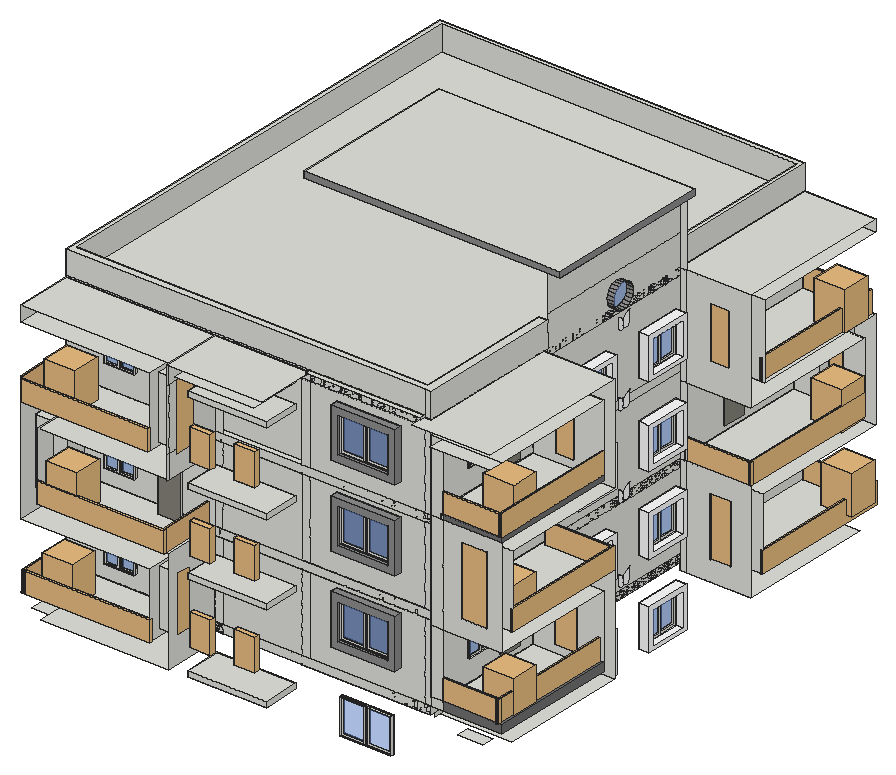
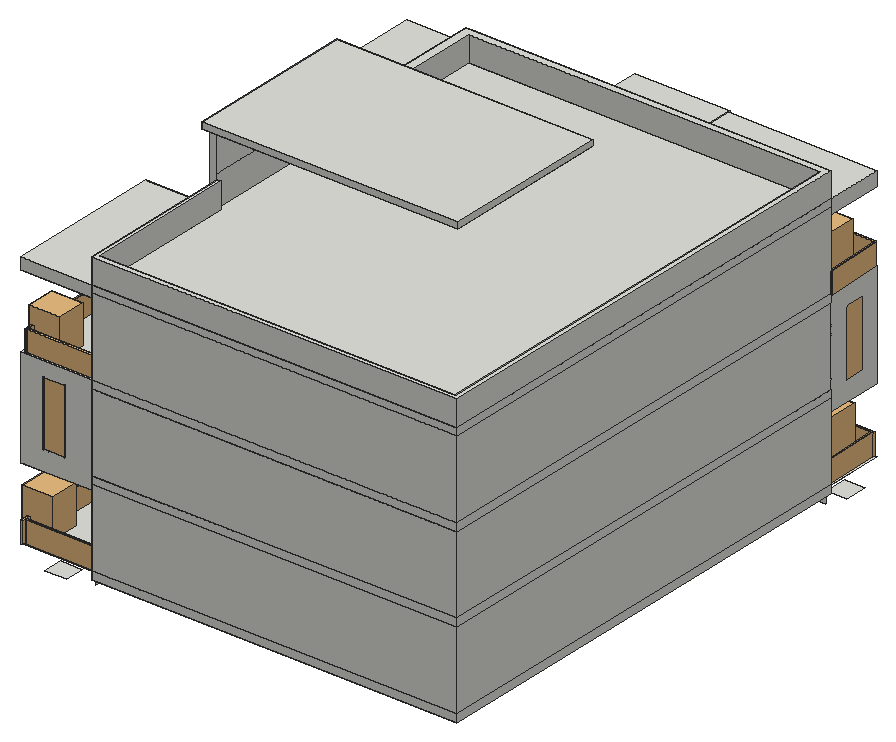
# SketchUp Ruby script. Lengths in inches.
U = 1.inch
M = Sketchup.active_model
def pt(a) = Geom::Point3d.new(a.map { |v| v * U })
def face(e, loops, mat)
  f = e.add_face(loops[0].map { |a| pt(a) })
  loops[1..].each { |l| e.add_face(l.map { |a| pt(a) }).erase! }
  f.material = f.back_material = mat if mat
  f
end
# faces: each face lists its corners as indices into pts; further lists are holes
def faces(e, pts, list, mat = nil) = list.each { |f| face(e, (f[0].is_a?(Array) ? f : [f]).map { |l| l.map { |i| pts[i] } }, mat) }
# xy, xz, yz: faces in a plane at the given z, y or x. An outline is a flat list of corners, or four numbers for a rectangle; further outlines are holes
def ring(l) = l.size == 4 ? [[l[0], l[1]], [l[2], l[1]], [l[2], l[3]], [l[0], l[3]]] : l.each_slice(2).to_a
def flat(e, list, mat, &to3) = list.each { |f| face(e, (f[0].is_a?(Array) ? f : [f]).map { |l| ring(l).map { |u, v| to3.(u, v) } }, mat) }
def xy(e, z, list, mat = nil) = flat(e, list, mat) { |x, y| [x, y, z] }
def xz(e, y, list, mat = nil) = flat(e, list, mat) { |x, z| [x, y, z] }
def yz(e, x, list, mat = nil) = flat(e, list, mat) { |y, z| [x, y, z] }
def lines(e, pts, list) = list.each { |a, b| e.add_line(pt(pts[a]), pt(pts[b])) }
# prism: a flat outline (further loops are holes) pulled along v
def prism(e, loops, v, mat = nil)
  f = face(e, loops, mat); d = Geom::Vector3d.new(v.map { |x| x * U })
  f.pushpull(f.normal.samedirection?(d) ? d.length : -d.length)
end
def box(e, o, s, mat = nil) = prism(e, [[o, [o[0] + s[0], o[1], o[2]], [o[0] + s[0], o[1] + s[1], o[2]], [o[0], o[1] + s[1], o[2]]]], [0, 0, s[2]], mat)
def at(x, y, z, deg = 0) = Geom::Transformation.translation(pt([x, y, z])) * Geom::Transformation.rotation(ORIGIN, Z_AXIS, deg.degrees)
def axes(o, x, y, z) = Geom::Transformation.new([*x, 0, *y, 0, *z, 0, *pt(o).to_a, 1])
def part(name) = M.definitions.add(name)
# library, detail: a bought-in or finely detailed component or shape, given as its bounding box
def library(name, o, s) = part(name).tap { |d| box(d.entities, o, s) }
def detail(e, o, s) = box(e.add_group.entities, o, s)
def put(e, d, t, mat = nil) = e.add_instance(d, t).tap { |i| i.material = mat if mat }
def group(e, t, mat = nil) = e.add_group.tap { |g| g.transformation = t; g.material = mat if mat }.entities
root = M.entities
M.materials.add("[Color M00]").color = [255, 255, 255]
M.materials.add("[Color M04]").color = [142, 142, 142]
M.materials.add("[Color M05]").color = [114, 114, 114]
M.materials.add("[Translucent Glass Blue]").color = [100, 149, 237]
M.materials["[Translucent Glass Blue]"].alpha = 0.5
M.materials.add("pic").color = [134, 132, 121]
c1 = part("Group\#73")
xy(c1.entities,0,[[6.22,6.22,66.16,57.66]],"[Color M00]")
xy(c1.entities,0,[[[0,0,72.375,63.875],[6.22,6.22,66.16,57.66]]],"[Color M04]")
xy(c1.entities,16.6875,[[[0,0,72.375,63.875],[6.22,6.22,66.16,57.66]]],"[Color M00]")
xz(c1.entities,0,[[0,0,72.375,16.6875]],"[Color M00]")
xz(c1.entities,6.22,[[6.22,0,66.16,16.6875]],"[Color M00]")
xz(c1.entities,57.66,[[6.22,0,66.16,16.6875]],"[Color M04]")
xz(c1.entities,63.875,[[0,0,72.375,16.6875]],"[Color M00]")
yz(c1.entities,0,[[0,0,63.875,16.6875]],"[Color M00]")
yz(c1.entities,6.22,[[6.22,0,57.66,16.6875]],"[Color M00]")
yz(c1.entities,66.16,[[6.22,0,57.66,16.6875]],"[Color M00]")
yz(c1.entities,72.375,[[0,0,63.875,16.6875]],"[Color M00]")
c2 = part("Janela aluminio")
xy(c2.entities,0,[[0,0,47.24,1.57],[23.62,1.57,47.24,2.76],[0,2.76,25.98,3.9375],[0,3.9375,47.24,5.91]])
xy(c2.entities,43.31,[[0,0,47.24,1.57],[23.62,1.57,47.24,2.76],[0,2.76,0,5.91,47.24,5.91,47.24,3.9375,25.98,3.9375,25.98,2.76],[25.98,2.76,47.24,3.9375]])
xz(c2.entities,1.57,[[0,0,23.62,0,23.62,41.34,21.26,41.34,21.26,1.97,1.97,1.97,1.97,41.34,23.62,41.34,23.62,43.31,0,43.31],[[23.62,0,47.24,43.31],[25.7,1.97,45.28,41.34]]])
xz(c2.entities,2.76,[[[0,0,23.62,43.31],[2.36,2.36,21.26,40.94]],[23.62,0,25.98,43.31]])
xz(c2.entities,2.76,[[2.36,2.36,21.26,40.94]],"[Translucent Glass Blue]")
xz(c2.entities,3.9375,[[25.98,0,25.98,2.36,44.88,2.36,44.88,40.94,25.98,40.94,25.98,43.31,47.24,43.31,47.24,0]])
xz(c2.entities,3.9375,[[25.98,2.36,44.88,40.94]],"[Translucent Glass Blue]")
yz(c2.entities,0,[[0,0,1.57,43.31],[2.76,0,5.91,43.31]])
yz(c2.entities,23.62,[[1.57,0,2.76,43.31]])
yz(c2.entities,25.98,[[2.76,0,3.9375,43.31]])
yz(c2.entities,47.24,[[0,0,1.57,43.31],[1.57,0,2.76,43.31],[3.9375,0,5.91,43.31]])
c3 = library("grade+varanda",[25.2,-1.57,0],[92.91,3.14,40.94])
c4 = part("Door leaf")
xy(c4.entities,0,[[0,0,28.74,2]],"pic")
xy(c4.entities,75.2,[[0,0,28.74,2]],"pic")
xz(c4.entities,0,[[0,0,28.74,75.2]],"pic")
xz(c4.entities,2,[[0,0,28.74,75.2]],"pic")
yz(c4.entities,0,[[0,0,2,75.2]])
yz(c4.entities,28.74,[[0,0,2,75.2]])
c5 = library("KentiaPalm",[-22.86,-14.31,0],[47.49,43.96,59.125])
c6 = library("Framed window",[0,0,0],[23.62,8.27,35.43])
c7 = library("CNC CUTTING TEXTURE",[0,0,-0.79],[85.98,295.47,0.79])
c8 = part("Group\#81")
xy(c8.entities,0,[[[0,0,99.375,76.3125],[10.74,10.74,88.63,65.57]],[10.74,10.74,88.63,65.57]])
xy(c8.entities,11.8125,[[[0,0,99.375,76.3125],[10.74,10.74,88.63,65.57]]])
xz(c8.entities,0,[[0,0,99.375,11.8125]])
xz(c8.entities,10.74,[[10.74,0,88.63,11.8125]])
xz(c8.entities,65.57,[[10.74,0,88.63,11.8125]])
xz(c8.entities,76.3125,[[0,0,99.375,11.8125]])
yz(c8.entities,0,[[0,0,76.3125,11.8125]])
yz(c8.entities,10.74,[[10.74,0,65.57,11.8125]])
yz(c8.entities,88.63,[[10.74,0,65.57,11.8125]])
yz(c8.entities,99.375,[[0,0,76.3125,11.8125]])
xy(root,534.42,[[206.95,156.57,237.95,190.94]])
xy(root,538.83,[[237.95,133.63,435.45,222.13]])
xy(root,541.5625,[[810.64,222.13,849.77,242.1]])
xy(root,541.92,[[809.28,913.11,842.4,942.88]])
xy(root,545.21,[[769.63,702.13,879.32,913.11]])
xy(root,548.14,[[769.63,242.1,879.32,439.19]])
xy(root,555.08,[[[206.95,222.13,769.63,942.88],[298.63,231.13,760.63,693.13]]])
xy(root,567.08,[[206.95,133.63,406.86,222.13],[[206.95,222.13,769.63,942.88],[298.63,231.13,760.63,693.13]],[769.63,222.13,879.32,222.13,879.32,418.66,867.32,418.66,867.32,232.68,769.63,232.68],[298.63,231.13,760.63,693.13],[769.63,232.68,867.32,418.66],
  [769.63,725.74,879.32,942.88]])
xy(root,576.07,[[815.46,702.13,848.03,725.74]])
xy(root,579.02,[[406.86,150.36,435.45,174.61]])
xy(root,579.0625,[[804.5,418.66,837.8125,439.19]])
xy(root,580.21,[[769.63,222.13,879.32,222.13,879.32,418.66,867.32,418.66,867.32,232.68,769.63,232.68]],"[Color M05]")
xy(root,665.39,[[406.86,150.36,435.45,174.61]])
xy(root,666.125,[[804.5,418.66,837.8125,439.19]])
xy(root,667.96,[[206.95,133.63,406.86,222.13]])
xy(root,668.01,[[815.46,702.13,848.03,725.74]])
xy(root,678.39,[[769.63,725.74,879.32,942.88]])
xy(root,679.46,[[769.63,222.13,879.32,418.66]])
xy(root,687.08,[[[206.95,222.13,769.63,942.88],[298.63,231.13,760.63,693.13]]])
xy(root,699.08,[[234.54,133.63,435.45,222.13],[[206.95,222.13,769.63,942.88],[298.63,231.13,760.63,693.13]],[298.63,231.13,760.63,693.13],[769.63,242.375,879.32,439.19],[769.63,702.13,879.32,921.54]])
xy(root,699.81,[[206.95,162.07,234.54,191.07]])
xy(root,705.14,[[816.88,222.13,856.51,242.375]])
xy(root,708.56,[[811.15,921.54,845.27,942.88]])
xy(root,800.75,[[206.95,162.07,234.54,191.07]])
xy(root,802.33,[[234.54,133.63,436.38,222.13]])
xy(root,807.39,[[769.63,702.13,879.32,921.54]])
xy(root,809.06,[[811.15,921.54,845.27,942.88]])
xy(root,811.33,[[816.88,222.13,856.51,242.375]])
xy(root,812.14,[[769.63,242.375,879.32,439.19]])
xy(root,819.08,[[[206.95,222.13,769.63,942.88],[298.63,231.13,760.63,693.13]]])
xy(root,831.08,[[206.95,133.63,406.75,222.13],[[206.95,222.13,769.63,942.88],[298.63,231.13,760.63,693.13]],[769.63,222.13,785.31,222.13,785.31,228.98,869.68,228.98,869.68,419.01,769.63,419.01],[785.31,222.13,879.32,222.13,879.32,419.01,869.68,419.01,869.68,228.98,785.31,228.98],[298.63,231.13,760.63,693.13],
  [769.63,728.37,879.32,942.88]])
xy(root,837.94,[[406.75,148.46,436.38,176.58]])
xy(root,839.08,[[785.31,222.13,879.32,222.13,879.32,419.01,869.68,419.01,869.68,228.98,785.31,228.98]],"[Color M05]")
xy(root,843.83,[[806.52,419.01,832.83,439.19]])
xy(root,849.98,[[817.23,702.13,844.91,728.37]])
xy(root,926.65,[[806.52,419.01,832.83,439.19]])
xy(root,929.29,[[817.23,702.13,844.91,728.37]])
xy(root,933.69,[[406.75,148.46,436.38,176.58]])
xy(root,939.77,[[206.95,133.63,406.75,222.13]])
xy(root,942.33,[[787.51,198.76,879.32,222.13],[769.63,222.13,879.32,419.01]])
xy(root,944.96,[[769.63,728.37,879.32,942.88]])
xy(root,951.08,[[448.85,129.69,571.01,157.26],[[206.95,222.13,769.63,942.88],[298.63,231.13,760.63,693.13]]])
xy(root,963.08,[[436.38,129.69,582.45,222.13],[206.95,133.63,436.38,222.13],[759.63,198.76,879.32,198.76,879.32,439.19,769.63,439.19,769.63,222.13,759.63,222.13],[206.95,222.13,206.95,942.88,769.63,942.88,769.63,702.13,763.98,702.13,763.98,935.9,214.93,935.9,214.93,233.34,755.82,233.34,755.82,222.13],[769.63,702.13,879.32,942.88]])
xy(root,966.02,[[582.45,214.57,759.63,222.13]])
xy(root,1001.83,[[206.95,222.13,769.63,222.13,769.63,447.18,755.82,447.18,755.82,233.34,214.93,233.34,214.93,935.9,763.98,935.9,763.98,702.13,769.63,702.13,769.63,942.88,206.95,942.88]])
xy(root,1067.71,[[394.95,447.18,769.63,702.13],[769.63,447.18,780.63,702.13],[394.95,702.13,789.63,706.38]])
xy(root,1067.71,[[394.95,445.74,789.63,447.18],[780.63,447.18,789.63,702.13]],"[Color M04]")
xy(root,1076.89,[[394.95,445.74,789.63,706.38]])
xz(root,148.46,[[406.75,837.94,436.38,933.69]])
xz(root,150.36,[[406.86,579.02,435.45,665.39]])
xz(root,162.07,[[206.95,699.81,234.54,800.75]])
xz(root,174.61,[[406.86,579.02,435.45,665.39]])
xz(root,176.58,[[406.75,837.94,436.38,933.69]])
xz(root,191.07,[[206.95,699.81,234.54,800.75]])
xz(root,222.13,[[213.89,538.83,435.45,555.08],[206.95,555.08,435.45,567.08],[436.38,555.08,448.85,567.08],[571.01,555.08,582.45,567.08],[582.45,555.08,759.63,567.08],
  [759.63,555.08,769.63,567.08],[206.95,567.08,406.86,667.96],[406.86,567.08,435.45,567.08,435.45,687.08,426.61,687.08,426.61,667.96,406.86,667.96],[435.45,567.08,436.38,687.08],[436.38,567.08,448.85,687.08],
  [448.85,567.08,571.01,687.08],[571.01,567.08,582.45,687.08],[582.45,567.08,759.63,687.08],[759.63,567.08,769.63,687.08],[769.63,567.08,787.51,580.21],
  [769.63,580.21,787.51,679.46],[206.95,667.96,426.61,687.08],[769.63,679.46,787.51,831.08],[[787.51,679.46,879.32,831.08],[816.88,705.14,856.51,811.33]],[206.95,687.08,435.45,699.08],
  [436.38,687.08,448.85,699.08],[571.01,687.08,582.45,699.08],[582.45,687.08,759.63,699.08],[759.63,687.08,769.63,699.08],[206.95,699.08,234.54,699.08,234.54,802.33,219.35,802.33,219.35,819.08,206.95,819.08],
  [234.54,699.08,436.38,802.33],[436.38,699.08,448.85,819.08],[448.85,699.08,571.01,819.08],[571.01,699.08,582.45,819.08],[582.45,699.08,759.63,819.08],
  [759.63,699.08,769.63,819.08],[219.35,802.33,436.38,819.08],[206.95,819.08,436.38,831.08],[436.38,819.08,448.85,831.08],[571.01,819.08,582.45,831.08],
  [582.45,819.08,759.63,831.08],[759.63,819.08,769.63,831.08],[206.95,831.08,406.75,939.77],[406.75,831.08,436.38,831.08,436.38,951.08,426.13,951.08,426.13,939.77,406.75,939.77],[436.38,831.08,448.85,951.08],
  [571.01,831.08,582.45,951.08],[582.45,831.08,759.63,951.08],[759.63,831.08,769.63,951.08],[769.63,831.08,769.63,942.33,787.51,942.33,787.51,839.08,785.31,839.08,785.31,831.08],[785.31,831.08,787.51,839.08],
  [206.95,939.77,426.13,951.08],[206.95,951.08,436.38,963.08],[436.38,951.08,582.45,963.08],[582.45,951.08,759.63,963.08],[759.63,951.08,769.63,963.08],
  [206.95,963.08,582.45,966.02],[582.45,963.08,759.63,966.02],[759.63,963.08,769.63,1001.83],[206.95,966.02,759.63,1001.83]])
xz(root,222.13,[[787.51,567.08,879.32,580.21],[787.51,831.08,879.32,839.08]],"[Color M05]")
xz(root,228.98,[[785.31,831.08,869.68,839.08]])
xz(root,231.13,[[298.63,567.08,760.63,687.08],[298.63,699.08,760.63,819.08],[298.63,831.08,760.63,951.08]])
xz(root,232.68,[[769.63,567.08,867.32,580.21]],"[Color M05]")
xz(root,233.34,[[214.93,963.08,755.82,1001.83]])
xz(root,242.375,[[[769.63,699.08,879.32,812.14],[816.88,705.14,856.51,811.33]]])
xz(root,418.66,[[[769.63,567.08,867.32,567.08,867.32,580.21,879.32,580.21,879.32,679.46,769.63,679.46],[804.5,579.0625,837.8125,666.125]],[867.32,567.08,879.32,580.21]])
xz(root,419.01,[[[769.63,831.08,869.68,831.08,869.68,839.08,879.32,839.08,879.32,942.33,769.63,942.33],[806.52,843.83,832.83,926.65]],[869.68,831.08,879.32,839.08]])
xz(root,439.19,[[[769.63,548.14,879.32,699.08],[804.5,579.0625,837.8125,666.125]],[[769.63,812.14,879.32,963.08],[806.52,843.83,832.83,926.65]]])
xz(root,445.74,[[394.95,1067.71,789.63,1076.89]],"[Color M04]")
xz(root,447.18,[[755.82,963.08,769.63,1001.83]])
xz(root,693.13,[[298.63,567.08,760.63,687.08],[298.63,699.08,760.63,819.08],[298.63,831.08,760.63,951.08]])
xz(root,702.13,[[769.63,545.21,780.63,699.08],[[780.63,545.21,879.32,699.08],[815.46,576.07,848.03,668.01]],[769.63,699.08,780.63,807.39],[769.63,807.39,780.63,963.08],[[780.63,807.39,879.32,963.08],[817.23,849.98,844.91,929.29]],
  [763.98,963.08,769.63,1001.83],[769.63,963.08,780.63,1067.71]])
xz(root,706.38,[[394.95,1067.71,789.63,1076.89]])
xz(root,725.74,[[[769.63,567.08,879.32,678.39],[815.46,576.07,848.03,668.01]]])
xz(root,728.37,[[[769.63,831.08,879.32,944.96],[817.23,849.98,844.91,929.29]]])
xz(root,921.54,[[769.63,699.08,879.32,699.08,879.32,807.39,845.27,807.39,845.27,708.56,811.15,708.56,811.15,807.39,769.63,807.39],[811.15,807.39,845.27,809.06]])
xz(root,935.9,[[214.93,963.08,763.98,1001.83]])
xz(root,942.88,[[206.95,567.08,769.63,687.08],[[769.63,678.39,879.32,831.08],[811.15,708.56,845.27,809.06]],[206.95,699.08,769.63,819.08],[206.95,831.08,769.63,951.08],[769.63,944.96,879.32,963.08],
  [206.95,963.08,769.63,1001.83]])
yz(root,206.95,[[222.13,567.08,942.88,687.08],[[133.63,667.96,222.13,831.08],[162.07,699.81,191.07,800.75]],[222.13,699.08,942.88,819.08],[222.13,831.08,942.88,951.08],[133.63,939.77,222.13,963.08],
  [222.13,963.08,942.88,1001.83]])
yz(root,214.93,[[233.34,963.08,935.9,1001.83]])
yz(root,234.54,[[[133.63,699.08,222.13,802.33],[162.07,699.81,191.07,800.75]]])
yz(root,298.63,[[231.13,567.08,693.13,687.08],[231.13,699.08,693.13,819.08],[231.13,831.08,693.13,951.08]])
yz(root,394.95,[[445.74,1067.71,706.38,1076.89]])
yz(root,406.75,[[[133.63,831.08,222.13,939.77],[148.46,837.94,176.58,933.69]]])
yz(root,406.86,[[[133.63,567.08,222.13,667.96],[150.36,579.02,174.61,665.39]]])
yz(root,435.45,[[[133.63,538.83,222.13,699.08],[150.36,579.02,174.61,665.39]]])
yz(root,436.38,[[129.69,802.33,133.63,837.94],[133.63,802.33,222.13,802.33,222.13,963.08,133.63,963.08,133.63,933.69,176.58,933.69,176.58,837.94,133.63,837.94],[129.69,837.94,133.63,933.69],[133.63,837.94,148.46,933.69],[148.46,837.94,176.58,933.69],
  [129.69,933.69,133.63,963.08]])
yz(root,582.45,[[214.57,963.08,222.13,966.02]])
yz(root,755.82,[[233.34,963.08,447.18,1001.83]])
yz(root,759.63,[[214.57,963.08,222.13,966.02]])
yz(root,760.63,[[231.13,567.08,693.13,687.08],[231.13,699.08,693.13,819.08],[231.13,831.08,693.13,951.08]])
yz(root,763.98,[[702.13,963.08,935.9,1001.83]])
yz(root,769.63,[[702.13,545.21,936.3,555.08],[230.73,548.14,439.19,555.08],[222.13,555.08,439.19,567.08],[447.18,555.08,702.13,567.08],[702.13,555.08,942.88,567.08],
  [232.68,567.08,418.66,567.08,418.66,679.46,222.13,679.46,222.13,580.21,232.68,580.21],[418.66,567.08,439.19,687.08],[439.19,567.08,447.18,687.08],[447.18,567.08,702.13,687.08],[702.13,567.08,725.74,567.08,725.74,678.39,709.31,678.39,709.31,687.08,702.13,687.08],
  [725.74,567.08,942.88,678.39],[709.31,678.39,942.88,687.08],[222.13,679.46,233.4375,687.08],[233.4375,679.46,418.66,687.08],[222.13,687.08,439.19,699.08],
  [447.18,687.08,702.13,699.08],[702.13,687.08,942.88,699.08],[222.13,699.08,242.375,819.08],[242.375,699.08,447.18,699.08,447.18,819.08,439.19,819.08,439.19,812.14,242.375,812.14],[447.18,699.08,702.13,819.08],
  [702.13,699.08,921.54,807.39],[921.54,699.08,942.88,699.08,942.88,819.08,935.42,819.08,935.42,807.39,921.54,807.39],[702.13,807.39,935.42,819.08],[242.375,812.14,421.32,819.08],[421.32,812.14,439.19,819.08],
  [222.13,819.08,439.19,831.08],[447.18,819.08,702.13,831.08],[702.13,819.08,942.88,831.08],[222.13,831.08,419.01,942.33],[419.01,831.08,439.19,831.08,439.19,951.08,421.32,951.08,421.32,942.33,419.01,942.33],
  [439.19,831.08,447.18,951.08],[447.18,831.08,702.13,951.08],[702.13,831.08,728.37,831.08,728.37,944.96,729.12,944.96,729.12,951.08,702.13,951.08],[728.37,831.08,942.88,944.96],[222.13,942.33,421.32,951.08],
  [729.12,944.96,942.88,951.08],[222.13,951.08,439.19,963.08],[447.18,951.08,702.13,1010.52],[702.13,951.08,942.88,963.08],[222.13,963.08,447.18,1001.83],
  [702.13,963.08,942.88,1001.83],[447.18,1010.52,702.13,1067.71]])
yz(root,770.82,[[579.22,962.375,584.15,962.9,588.78,964.6875,592.79,967.61,595.9,971.47,597.91,976,598.68,980.9,598.15,985.84,596.36,990.46,593.44,994.47,589.58,997.59,585.05,999.6,580.15,1000.36,575.22,999.84,570.59,998.05,566.58,995.13,563.47,991.27,561.46,986.73,560.6875,981.83,561.22,976.9,563,972.27,565.92,968.27,569.78,965.15,574.32,963.14]],"[Translucent Glass Blue]")
yz(root,780.63,[[577.58,580.375,578.17,580.9,578.83,581.44,579.23,582.16,579.45,582.99,579.62,583.85,578.67,585.9,578.48,586.67,578.04,587.35,578.04,588.17,578.03,589.07,577.98,589.875,577.92,590.85,577.81,591.61,577.48,592.37,577.16,593.04,576.92,593.91,576.64,594.73,576.3,595.43,575.73,596.1,575.21,596.56,574.43,597.22,573.76,597.85,572.95,598.14,572.6875,598.71,571.06,599.29,571,597.42,571.5,595.73,571.63,594.04,571.52,593.42,571.55,592.62,571.54,591.77,571.52,591.01,571.5,590.24,571.36,589.13,571.1,588.42,571.01,587.41,570.9375,586.58,570.87,585.67,571.05,584.95,571.28,584.18,571.66,583.4,572.09,582.51,572.79,582.05,573.44,581.44,574.125,580.95,574.95,580.73,575.7,580.57,576.67,580.45],[587.71,581.05,588.31,581.6,588.74,582.28,589.32,582.92,589.55,583.75,589.71,584.62,589.84,585.63,589.91,586.46,589.97,587.39,590.01,588.44,590.04,589.29,590.07,590.22,590.09,591.17,590.11,591.88,590.13,592.66,590.03,593.44,590.03,594.2,589.7,595.2,589.63,596.12,589.59,596.93,589.56,597.85,589.55,598.77,589.56,599.6875,589.65,600.27,589.35,600.01,588.79,599.95,588.13,599.5625,587.47,599.03,586.76,598.66,586.15,598.16,585.43,597.75,584.71,597.25,583.98,596.84,583.01,596.11,582.55,595.42,581.94,594.94,581.45,594.26,581.12,593.55,580.71,592.85,580.42,592,580.27,591.12,580.16,590.22,579.97,589.3,579.89,588.37,579.83,587.66,579.78,586.88,579.62,583.85,581.3,582.31,582.77,581.32,584.45,581.1,584.98,581.22,585.85,581.11,586.81,581.07],[577.58,697.5,578.17,698.03,578.83,698.56,579.23,699.29,579.45,700.11,579.62,700.97,578.67,703.03,578.48,703.8,578.04,704.48,578.04,705.29,578.03,706.2,577.98,707,577.92,707.97,577.81,708.73,577.48,709.49,577.16,710.16,576.92,711.03,576.64,711.85,576.3,712.55,575.73,713.23,575.21,713.68,574.43,714.35,573.76,714.98,572.95,715.27,572.6875,715.83,571.06,716.41,571,714.54,571.5,712.85,571.63,711.16,571.52,710.54,571.55,709.74,571.54,708.9,571.52,708.14,571.5,707.37,571.36,706.26,571.1,705.55,571.01,704.54,570.9375,703.7,570.87,702.79,571.05,702.08,571.28,701.3,571.66,700.52,572.09,699.64,572.79,699.18,573.44,698.57,574.125,698.07,574.95,697.86,575.7,697.69,576.67,697.57],[587.71,698.18,588.31,698.73,588.74,699.41,589.32,700.05,589.55,700.875,589.71,701.75,589.84,702.76,589.91,703.59,589.97,704.51,590.01,705.57,590.04,706.41,590.07,707.35,590.09,708.3,590.11,709,590.13,709.79,590.03,710.57,590.03,711.33,589.7,712.32,589.63,713.24,589.59,714.05,589.56,714.97,589.55,715.89,589.56,716.8125,589.65,717.39,589.35,717.14,588.79,717.07,588.13,716.6875,587.47,716.16,586.76,715.79,586.15,715.28,585.43,714.875,584.71,714.37,583.98,713.96,583.01,713.23,582.55,712.54,581.94,712.07,581.45,711.38,581.12,710.68,580.71,709.97,580.42,709.125,580.27,708.25,580.16,707.35,579.97,706.43,579.89,705.5,579.83,704.79,579.78,704,579.62,700.97,581.3,699.43,582.77,698.45,584.45,698.22,584.98,698.34,585.85,698.24,586.81,698.19],[577.58,824.8125,578.17,825.34,578.83,825.88,579.23,826.6,579.45,827.42,579.62,828.29,578.67,830.34,578.48,831.11,578.04,831.79,578.04,832.61,578.03,833.51,577.98,834.3125,577.92,835.29,577.81,836.05,577.48,836.81,577.16,837.48,576.92,838.34,576.64,839.16,576.3,839.86,575.73,840.54,575.21,840.99,574.43,841.66,573.76,842.29,572.95,842.58,572.6875,843.14,571.06,843.72,571,841.86,571.5,840.17,571.63,838.48,571.52,837.85,571.55,837.05,571.54,836.21,571.52,835.45,571.5,834.68,571.36,833.57,571.1,832.86,571.01,831.85,570.9375,831.01,570.87,830.1,571.05,829.39,571.28,828.61,571.66,827.83,572.09,826.95,572.79,826.49,573.44,825.88,574.125,825.39,574.95,825.17,575.7,825.01,576.67,824.89],
  [587.71,825.49,588.31,826.04,588.74,826.72,589.32,827.36,589.55,828.1875,589.71,829.06,589.84,830.07,589.91,830.9,589.97,831.82,590.01,832.88,590.04,833.72,590.07,834.66,590.09,835.61,590.11,836.32,590.13,837.1,590.03,837.88,590.03,838.64,589.7,839.63,589.63,840.55,589.59,841.36,589.56,842.28,589.55,843.21,589.56,844.125,589.65,844.7,589.35,844.45,588.79,844.38,588.13,844,587.47,843.47,586.76,843.1,586.15,842.6,585.43,842.1875,584.71,841.68,583.98,841.27,583.01,840.54,582.55,839.85,581.94,839.38,581.45,838.7,581.12,837.99,580.71,837.28,580.42,836.4375,580.27,835.56,580.16,834.66,579.97,833.74,579.89,832.81,579.83,832.1,579.78,831.32,579.62,828.29,581.3,826.75,582.77,825.76,584.45,825.53,584.98,825.66,585.85,825.55,586.81,825.51],[577.58,936.0625,578.17,936.59,578.83,937.13,579.23,937.85,579.45,938.67,579.62,939.54,578.67,941.59,578.48,942.36,578.04,943.04,578.04,943.86,578.03,944.76,577.98,945.5625,577.92,946.54,577.81,947.3,577.48,948.06,577.16,948.73,576.92,949.59,576.64,950.41,576.3,951.11,575.73,951.79,575.21,952.24,574.43,952.91,573.76,953.54,572.95,953.83,572.6875,954.39,571.06,954.97,571,953.11,571.5,951.42,571.63,949.73,571.52,949.1,571.55,948.3,571.54,947.46,571.52,946.7,571.5,945.93,571.36,944.82,571.1,944.11,571.01,943.1,570.9375,942.26,570.87,941.35,571.05,940.64,571.28,939.86,571.66,939.08,572.09,938.2,572.79,937.74,573.44,937.13,574.125,936.64,574.95,936.42,575.7,936.26,576.67,936.14],[587.71,936.74,588.31,937.29,588.74,937.97,589.32,938.61,589.55,939.4375,589.71,940.31,589.84,941.32,589.91,942.15,589.97,943.07,590.01,944.13,590.04,944.97,590.07,945.91,590.09,946.86,590.11,947.57,590.13,948.35,590.03,949.13,590.03,949.89,589.7,950.88,589.63,951.8,589.59,952.61,589.56,953.53,589.55,954.46,589.56,955.375,589.65,955.95,589.35,955.7,588.79,955.63,588.13,955.25,587.47,954.72,586.76,954.35,586.15,953.85,585.43,953.4375,584.71,952.93,583.98,952.52,583.01,951.79,582.55,951.1,581.94,950.63,581.45,949.95,581.12,949.24,580.71,948.53,580.42,947.6875,580.27,946.81,580.16,945.91,579.97,944.99,579.89,944.06,579.83,943.35,579.78,942.57,579.62,939.54,581.3,938,582.77,937.01,584.45,936.78,584.98,936.91,585.85,936.8,586.81,936.76]],"[Color M00]")
yz(root,780.63,[[589.65,600.27,590.67,601.13,591.45,602.62,589.67,600.39],[589.65,717.39,590.67,718.25,591.45,719.75,589.67,717.52],[589.65,844.7,590.67,845.57,591.45,847.06,589.67,844.83],[589.65,955.95,590.67,956.82,591.45,958.31,589.67,956.08]],"[Color M04]")
yz(root,785.31,[[222.13,831.08,228.98,839.08]])
yz(root,789.63,[[445.74,1067.71,706.38,1076.89]],"[Color M04]")
yz(root,804.5,[[418.66,579.0625,439.19,666.125]])
yz(root,806.52,[[419.01,843.83,439.19,926.65]])
yz(root,811.15,[[921.54,708.56,942.88,809.06]])
yz(root,815.46,[[702.13,576.07,725.74,668.01]])
yz(root,816.88,[[222.13,705.14,242.375,811.33]])
yz(root,817.23,[[702.13,849.98,728.37,929.29]])
yz(root,832.83,[[419.01,843.83,439.19,926.65]])
yz(root,837.8125,[[418.66,579.0625,439.19,666.125]])
yz(root,844.91,[[702.13,849.98,728.37,929.29]])
yz(root,845.27,[[921.54,708.56,942.88,809.06]])
yz(root,848.03,[[702.13,576.07,725.74,668.01]])
yz(root,856.51,[[222.13,705.14,242.375,811.33]])
yz(root,867.32,[[232.68,567.08,418.66,580.21]],"[Color M05]")
yz(root,869.68,[[228.98,831.08,419.01,839.08]],"[Color M05]")
yz(root,879.32,[[222.13,567.08,418.66,580.21],[222.13,831.08,419.01,839.08]],"[Color M05]")
p = [[780.63,574.32,963.14],[780.63,579.22,962.375],[770.82,579.22,962.375],[770.82,574.32,963.14],[780.63,584.15,962.9],[770.82,584.15,962.9],
  [780.63,588.78,964.6875],[770.82,588.78,964.6875],[780.63,569.78,965.15],[770.82,569.78,965.15],[780.63,592.79,967.61],[770.82,592.79,967.61],
  [780.63,565.92,968.27],[770.82,565.92,968.27],[780.63,595.9,971.47],[770.82,595.9,971.47],[780.63,563,972.27],[770.82,563,972.27],
  [780.63,597.91,976],[770.82,597.91,976],[780.63,561.22,976.9],[770.82,561.22,976.9],[780.63,598.68,980.9],[770.82,598.68,980.9],
  [780.63,560.6875,981.83],[770.82,560.6875,981.83],[780.63,598.15,985.84],[770.82,598.15,985.84],[780.63,561.46,986.73],[770.82,561.46,986.73],
  [780.63,596.36,990.46],[770.82,596.36,990.46],[780.63,563.47,991.27],[770.82,563.47,991.27],[780.63,593.44,994.47],[770.82,593.44,994.47],
  [780.63,566.58,995.13],[770.82,566.58,995.13],[780.63,589.58,997.59],[770.82,589.58,997.59],[780.63,570.59,998.05],[770.82,570.59,998.05],
  [780.63,585.05,999.6],[770.82,585.05,999.6],[780.63,575.22,999.84],[770.82,575.22,999.84],[780.63,580.15,1000.36],[770.82,580.15,1000.36],
  [780.63,578.67,941.59],[780.63,579.08,940.9375],[780.63,569.41,954.99],[780.63,571.06,954.97],[780.63,578.67,830.34],[780.63,579.08,829.6875],
  [780.63,569.41,843.74],[780.63,571.06,843.72],[780.63,578.67,703.03],[780.63,579.08,702.375],[780.63,569.41,716.43],[780.63,571.06,716.41],
  [780.63,578.67,585.9],[780.63,579.08,585.25],[780.63,569.41,599.31],[780.63,571.06,599.29],[571.01,210.63,951.08],[571.01,157.26,951.08]]
faces(root,p,[[0,1,2,3],[1,4,5,2],[4,6,7,5],[8,0,3,9],[6,10,11,7],[12,8,9,13],[10,14,15,11],[16,12,13,17],
  [14,18,19,15],[20,16,17,21],[18,22,23,19],[24,20,21,25],[22,26,27,23],[28,24,25,29],[26,30,31,27],[32,28,29,33],
  [30,34,35,31],[36,32,33,37],[34,38,39,35],[40,36,37,41],[38,42,43,39],[44,40,41,45],[42,46,47,43],[46,44,45,47]],"[Color M04]")
lines(root,p,[[48,49],[50,51],[52,53],[54,55],[56,57],[58,59],[60,61],[62,63],[64,65]])
put(root,c1,axes([780.82,472.87,478.49],[0,1,0],[0,0,1],[1,0,0]),"[Color M00]")
put(root,c1,axes([780.63,608.66,480.34],[0,1,0],[0,0,1],[1,0,0]),"[Color M00]")
put(root,c2,axes([785.51,479.08,484.46],[0,1.25,0],[-1,0,0],[0,0,1.1998]))
put(root,c2,axes([786.92,614.88,486.5625],[0,1.25,0],[-1,0,0],[0,0,1.1998]))
put(root,c2,axes([720.02,213.44,487.69],[-1.675,0,0],[0,-1,0],[0,0,1.25072]))
g1 = group(root,at(448.85,210.63,525.93))
box(g1,[0,-57.1875,0],[122.16,57.1875,8.15])
g2 = group(root,at(289.63,702.13,555.08))
box(g2,[-82.6875,-480,0],[562.6875,720.75,12])
put(root,c3,axes([157.3,134.04,566.47],[2.12,0,0],[0,1,0],[0,0,0.8]))
put(root,c3,axes([743.65,939.6,566.91],[1.0998,0,0],[0,1,0],[0,0,0.8]))
put(root,c3,axes([877.75,666.45,567.08],[0,2.3532,0],[-1,0,0],[0,0,0.8]))
put(root,c3,axes([209.39,244.3,567.08],[0.02789,-0.93959,0],[0.99956,0.02967,0],[0,0,0.8]))
put(root,c4,axes([360.64,220.13,567.08],[1.26,0,0],[0,1,0],[0,0,1.1]))
put(root,c5,at(850.68,263.55,570.92))
put(root,c5,at(261.29,149.54,571.6))
put(root,c4,axes([771.63,787.51,574.24],[0,1.26,0],[-1,0,0],[0,0,1.1]))
put(root,c6,axes([529.875,141.71,575.71],[1.35,0,0],[0,1,0],[0,0,1.38]))
put(root,c6,axes([461.6875,141.71,575.71],[1.35,0,0],[0,1,0],[0,0,1.38]))
put(root,c7,axes([817.49,702.13,576.07],[0.35511,0,0],[0,0,0.31122],[0,-7.22297,0]))
put(root,c4,axes([771.63,355.51,576.34],[0,1.26,0],[-1,0,0],[0,0,1.1]))
put(root,c7,axes([804.33,418.66,578.86],[0.3894,0,0],[0,0,0.29533],[0,-1.1913,0]))
put(root,c7,axes([429.51,150.36,579.02],[0,0.28203,0],[0,0,0.29233],[-6.34963,0,0]))
put(root,c5,at(863.69,900.52,579.08))
put(root,c3,axes([872.21,168.27,579.14],[0,2.12,0],[-1,0,0],[0,0,0.8]))
put(root,c3,axes([763.82,223.71,579.73],[0.94,0,0],[0,1,0],[0,0,0.8]))
put(root,c2,at(269.17,216.22,590.9))
put(root,c2,at(774.2,291.2,604.36,90))
put(root,c8,axes([630.14,214.57,609.22],[1,0,0],[0,0,1],[0,-1,0]),"[Color M04]")
put(root,c1,axes([780.63,608.66,610.09],[0,1,0],[0,0,1],[1,0,0]),"[Color M00]")
put(root,c1,axes([780.82,472.87,610.86],[0,1,0],[0,0,1],[1,0,0]),"[Color M00]")
put(root,c2,at(774.2,845.05,614.86,90))
put(root,c2,axes([786.92,614.88,616.3125],[0,1.25,0],[-1,0,0],[0,0,1.1998]))
put(root,c2,axes([785.51,479.08,617.08],[0,1.25,0],[-1,0,0],[0,0,1.1998]))
put(root,c2,axes([720.02,213.44,620.63],[-1.675,0,0],[0,-1,0],[0,0,1.25072]))
g3 = group(root,at(448.85,210.63,661.18))
box(g3,[0,-57.1875,0],[122.16,57.1875,8.15])
g4 = group(root,at(289.63,702.13,687.08))
box(g4,[-82.6875,-480,0],[562.6875,720.75,12])
put(root,c5,at(854.6875,891.35,695.82))
put(root,c3,axes([425.8125,244.5,697.97],[0.02789,-0.93959,0],[0.99956,0.02967,0],[0,0,0.8]))
put(root,c3,axes([746.74,436.94,698.71],[1.0998,0,0],[0,1,0],[0,0,0.8]))
put(root,c3,axes([181.12,132.06,698.9],[2.12,0,0],[0,1,0],[0,0,0.8]))
put(root,c3,axes([877.75,188.96,699.08],[0,2.12,0],[-1,0,0],[0,0,0.8]))
put(root,c5,at(850.68,263.81,699.08))
put(root,c3,axes([877.75,643.6,699.08],[0,2.3532,0],[-1,0,0],[0,0,0.8]))
put(root,c3,axes([749.5,703.75,699.08],[1.0998,0,0],[0,1,0],[0,0,0.8]))
put(root,c7,axes([207.88,162.07,699.25],[0,0.33727,0],[0,0,0.34352],[1.1913,0,0]))
put(root,c6,axes([529.875,141.71,702.27],[1.35,0,0],[0,1,0],[0,0,1.38]))
put(root,c6,axes([461.6875,141.71,702.27],[1.35,0,0],[0,1,0],[0,0,1.38]))
put(root,c5,at(270.46,146.21,703.31))
put(root,c4,axes([369.66,195.07,704.86],[1.26,0,0],[0,1,0],[0,0,1.1]))
put(root,c7,axes([816.88,222.13,705.14],[0.46084,0,0],[0,0,0.35938],[0,-1.1913,0]))
put(root,c4,axes([771.63,787.51,707.24],[0,1.26,0],[-1,0,0],[0,0,1.1]))
put(root,c7,axes([811.15,942.88,708.56],[0.38524,0,0],[0,0,0.34013],[0,6.12304,0]))
put(root,c4,axes([771.63,355.51,715.41],[0,1.26,0],[-1,0,0],[0,0,1.1]))
put(root,c2,at(269.17,216.22,723.49))
put(root,c1,axes([780.63,608.66,731.47],[0,1,0],[0,0,1],[1,0,0]),"[Color M00]")
put(root,c2,at(774.2,291.2,735.54,90))
put(root,c1,axes([780.82,472.87,735.98],[0,1,0],[0,0,1],[1,0,0]),"[Color M00]")
put(root,c2,axes([786.92,614.88,737.6875],[0,1.25,0],[-1,0,0],[0,0,1.1998]))
put(root,c8,axes([630.14,214.57,741.35],[1,0,0],[0,0,1],[0,-1,0]),"[Color M04]")
put(root,c2,axes([785.51,479.08,742.19],[0,1.25,0],[-1,0,0],[0,0,1.1998]))
put(root,c2,at(774.2,845.05,744.23,90))
put(root,c2,axes([720.02,213.44,752.75],[-1.675,0,0],[0,-1,0],[0,0,1.25072]))
g5 = group(root,at(448.85,210.63,785.24))
box(g5,[0,-57.1875,0],[122.16,57.1875,8.15])
g6 = group(root,at(289.63,702.13,819.08))
box(g6,[-82.6875,-480,0],[562.6875,720.75,12])
put(root,c3,axes([873.35,670.68,831.08],[0,2.2896,0],[-1,0,0],[0,0,0.8]))
put(root,c5,at(854.6875,898.32,831.08))
put(root,c3,axes([204.67,245.76,831.08],[0.02789,-0.93959,0],[0.99956,0.02967,0],[0,0,0.8]))
put(root,c3,axes([156.36,132.06,831.08],[2.12,0,0],[0,1,0],[0,0,0.8]))
put(root,c4,axes([341.91,220.13,831.24],[1.26,0,0],[0,1,0],[0,0,1.1]))
put(root,c6,axes([461.6875,141.71,831.89],[1.35,0,0],[0,1,0],[0,0,1.38]))
put(root,c6,axes([529.875,141.71,831.89],[1.35,0,0],[0,1,0],[0,0,1.38]))
put(root,c3,axes([743.65,939.6,832.16],[1.0998,0,0],[0,1,0],[0,0,0.8]))
put(root,c7,axes([437.32,148.46,832.19],[0,0.33727,0],[0,0,0.34352],[1.1913,0,0]))
put(root,c5,at(256.71,160.59,833.36))
put(root,c4,axes([771.63,355.51,834.78],[0,1.26,0],[-1,0,0],[0,0,1.1]))
put(root,c3,axes([763.82,223.71,837.67],[0.94,0,0],[0,1,0],[0,0,0.8]))
put(root,c5,at(850.68,263.55,838.54))
put(root,c3,axes([877.75,168.62,839.08],[0,2.12,0],[-1,0,0],[0,0,0.8]))
put(root,c4,axes([771.63,787.51,839.61],[0,1.26,0],[-1,0,0],[0,0,1.1]))
put(root,c7,axes([806.52,418.07,843.83],[0.30602,0,0],[0,0,0.29242],[0,-1.1913,0]))
put(root,c7,axes([817.23,706.95,849.98],[0.32201,0,0],[0,0,0.26843],[0,6.12304,0]))
put(root,c1,axes([780.63,608.66,855.28],[0,1,0],[0,0,1],[1,0,0]),"[Color M00]")
put(root,c1,axes([780.82,472.87,856.85],[0,1,0],[0,0,1],[1,0,0]),"[Color M00]")
put(root,c2,axes([786.92,614.88,861.5],[0,1.25,0],[-1,0,0],[0,0,1.1998]))
put(root,c2,axes([786.69,479.08,862.84],[0,1.25,0],[-1,0,0],[0,0,1.1998]))
put(root,c8,axes([630.14,214.57,867.03],[1,0,0],[0,0,1],[0,-1,0]),"[Color M04]")
put(root,c2,at(774.2,290.89,867.67,90))
put(root,c2,at(269.17,216.22,868.53))
put(root,c2,at(774.2,845.05,874.17,90))
put(root,c2,axes([720.02,213.44,878.43],[-1.675,0,0],[0,-1,0],[0,0,1.25072]))
g7 = group(root,at(448.85,210.63,912.43))
box(g7,[0,-57.1875,0],[122.16,57.1875,8.15])
g8 = group(root,at(289.63,702.13,951.08))
box(g8,[-82.6875,-480,0],[562.6875,720.75,12])
